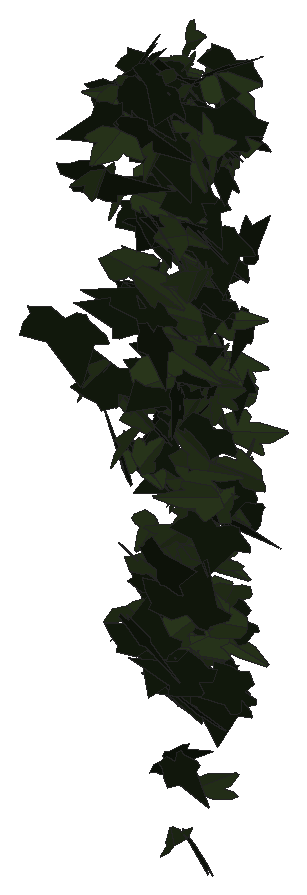
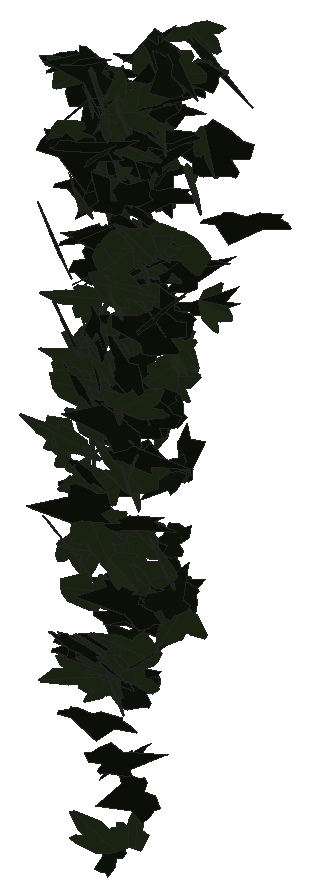
# SketchUp Ruby script. Lengths in millimetres.
U = 1.mm
M = Sketchup.active_model
def pt(a) = Geom::Point3d.new(a.map { |v| v * U })
def face(e, loops, mat)
  f = e.add_face(loops[0].map { |a| pt(a) })
  loops[1..].each { |l| e.add_face(l.map { |a| pt(a) }).erase! }
  f.material = f.back_material = mat if mat
  f
end
# faces: each face lists its corners as indices into pts; further lists are holes
def faces(e, pts, list, mat = nil) = list.each { |f| face(e, (f[0].is_a?(Array) ? f : [f]).map { |l| l.map { |i| pts[i] } }, mat) }
# xy, xz, yz: faces in a plane at the given z, y or x. An outline is a flat list of corners, or four numbers for a rectangle; further outlines are holes
def ring(l) = l.size == 4 ? [[l[0], l[1]], [l[2], l[1]], [l[2], l[3]], [l[0], l[3]]] : l.each_slice(2).to_a
def flat(e, list, mat, &to3) = list.each { |f| face(e, (f[0].is_a?(Array) ? f : [f]).map { |l| ring(l).map { |u, v| to3.(u, v) } }, mat) }
def xy(e, z, list, mat = nil) = flat(e, list, mat) { |x, y| [x, y, z] }
def xz(e, y, list, mat = nil) = flat(e, list, mat) { |x, z| [x, y, z] }
def yz(e, x, list, mat = nil) = flat(e, list, mat) { |y, z| [x, y, z] }
def lines(e, pts, list) = list.each { |a, b| e.add_line(pt(pts[a]), pt(pts[b])) }
# prism: a flat outline (further loops are holes) pulled along v
def prism(e, loops, v, mat = nil)
  f = face(e, loops, mat); d = Geom::Vector3d.new(v.map { |x| x * U })
  f.pushpull(f.normal.samedirection?(d) ? d.length : -d.length)
end
def box(e, o, s, mat = nil) = prism(e, [[o, [o[0] + s[0], o[1], o[2]], [o[0] + s[0], o[1] + s[1], o[2]], [o[0], o[1] + s[1], o[2]]]], [0, 0, s[2]], mat)
def at(x, y, z, deg = 0) = Geom::Transformation.translation(pt([x, y, z])) * Geom::Transformation.rotation(ORIGIN, Z_AXIS, deg.degrees)
def axes(o, x, y, z) = Geom::Transformation.new([*x, 0, *y, 0, *z, 0, *pt(o).to_a, 1])
def part(name) = M.definitions.add(name)
# library, detail: a bought-in or finely detailed component or shape, given as its bounding box
def library(name, o, s) = part(name).tap { |d| box(d.entities, o, s) }
def detail(e, o, s) = box(e.add_group.entities, o, s)
def put(e, d, t, mat = nil) = e.add_instance(d, t).tap { |i| i.material = mat if mat }
def group(e, t, mat = nil) = e.add_group.tap { |g| g.transformation = t; g.material = mat if mat }.entities
root = M.entities
M.materials.add("efeu1").color = [18, 25, 13]
M.materials.add("efeu2").color = [43, 57, 29]
c1 = part("ivyleaf_10")
p = [[0,12.8,-0.8],[-1.5,51.3,-10.9],[-4.9,51,-11.6],[-13.6,26.5,-7.3],[-13.2,15.9,-4.6],[-21.1,19.3,-7.2],
  [-29.5,16.3,-8.3],[-29.2,8.3,-6.2],[-19.7,-9.8,0.5],[-7.6,-13,4],[1,-12.2,5.8],[-0.4,51.1,-11.1],
  [-1.5,51.1,-10.9],[1,-12.4,5.9],[16.9,-12.4,3.5],[35.1,9.1,-5.1],[35,12.9,-6.1],[20.5,16.4,-4.9],
  [15.8,15,-3.8],[15.3,27.6,-7.1],[12.8,31.3,-7.8]]
faces(c1.entities,p,[[0,1,2,3,4,5,6,7,8,9,10],[11,12,0,13,14,15,16,17,18,19,20]],"efeu2")
c2 = part("ivyleaf_9")
p = [[39.1,54.8,31.7],[34.5,51.8,30.2],[-5.3,25.2,17.3],[-17.9,28.3,20.9],[-21.6,21.7,17],[-20.2,4.3,5.3],
  [-22.9,-0.3,2.5],[-17.1,-4,-0.6],[-2,-2.1,-1.2],[-0.7,-15.4,-10.1],[16.6,-22.3,-16.7],[21.1,-15.1,-12.5],
  [32.7,-10.7,-11],[46.1,-1.8,-6.6],[30.8,11.2,3.8]]
faces(c2.entities,p,[[0,1,2,3,4,5,6,7,8,9,10,11,12,13,14]],"efeu1")
put(root,c1,axes([3253.9,934.5,1390.3],[0.28843,0.04312,-0.8785],[1.25745,0.58285,0.14259],[1.10498,-0.67454,0.06705]))
put(root,c1,axes([3248.6,977.3,1386.9],[-0.36025,0.03868,0.8413],[1.53515,-0.23963,0.1925],[0.46091,0.82837,0.01641]))
put(root,c2,axes([3287.5,931.1,1234.8],[0.00435,-0.95208,0.10893],[0.11387,0.10886,0.95021],[-1.82026,0.00453,0.0597]))
put(root,c2,axes([3277.1,907.7,776.3],[1.0892,-0.78694,0.12747],[-0.13915,0.10444,0.97303],[-1.51082,-0.57695,0.00228]))
put(root,c1,axes([3291.6,962.2,1116.4],[1.27719,0.56046,0.4478],[-0.68997,-0.26417,0.87394],[1.17815,-0.76229,0.02637]))
put(root,c1,axes([3285.6,790.1,1475.8],[-0.46484,-1.03607,-0.08668],[0.02141,0.0864,-1.06443],[1.97862,-0.24434,-0.00884]))
put(root,c2,axes([3273,919,1588.6],[-0.4291,-0.87355,0.10052],[-0.05183,-0.09678,-0.90217],[1.67271,-0.22709,-0.00217]))
put(root,c2,axes([3281.5,876.4,1606.8],[0.34168,0.36068,0.93092],[0.51666,0.89258,-0.39818],[-1.82847,0.31961,0.06145]))
put(root,c2,axes([3265.6,884.9,987.3],[1.22662,-0.55899,-0.33011],[-0.47279,0.21739,-0.85315],[1.14149,0.69072,0.00136]))
put(root,c2,axes([3295.7,835.9,975.3],[0.02806,-0.50522,0.9314],[-0.00193,0.93148,0.50528],[-2.01663,-0.00792,0.01247]))
put(root,c1,axes([3299.6,879.7,1527.1],[-0.16158,0.22237,0.91702],[-1.11907,0.70764,-0.22604],[-1.40456,-0.58939,0.0746]))
put(root,c2,axes([3265.9,941.3,721.2],[0.65263,-0.85103,-0.29467],[-0.14747,0.28626,-0.91691],[1.70767,0.34997,0.03343]))
put(root,c1,axes([3287.3,900.9,857.4],[1.13215,-0.76866,-0.10225],[-0.11057,0.08433,-0.97195],[1.47166,0.59767,0.00564]))
put(root,c1,axes([3309.9,840.2,1594.3],[0.04476,0.06694,-1.05229],[-1.47456,-0.71285,-0.06266],[-1.36119,0.77442,0.03328]))
put(root,c2,axes([3311,992.6,552.1],[-0.28006,-0.04072,0.84102],[-1.52909,-0.24865,-0.15261],[0.47946,-0.81678,0.00453]))
put(root,c2,axes([3322.5,944.6,1028.3],[-1.09052,-0.28515,-0.64426],[-1.04808,-0.3367,0.6388],[-0.83635,0.79374,0.03953]))
put(root,c1,axes([3290.9,828.6,1425.4],[0.64577,-0.87683,-0.10025],[-0.03836,0.09968,-0.94004],[1.67922,0.33947,0.01708]))
put(root,c1,axes([3284.6,860.6,738.5],[-0.95757,-0.67439,-0.51289],[0.57513,0.41444,-0.84138],[1.50647,-0.58689,-0.0048]))
put(root,c2,axes([3274.9,887.2,1511.2],[-0.04256,-0.96485,-0.17622],[0.03285,0.17585,-0.96502],[1.86639,-0.0251,0.01297]))
put(root,c1,axes([3298.9,937.3,1019.6],[0.05472,0.6044,-0.66477],[-0.19068,0.66312,0.59856],[1.69927,0.05495,0.08858]))
put(root,c2,axes([3307.2,957.2,923.1],[-1.16527,-0.46556,0.47357],[-0.66857,-0.31958,-0.76835],[1.0726,-0.70499,0.03556]))
put(root,c1,axes([3296.2,821,1591],[0.65116,0.6651,-0.58723],[-0.60239,-0.49647,-0.74672],[-1.57749,0.46413,0.04275]))
put(root,c2,axes([3293.1,893.4,1564.3],[-1.0739,-0.73088,-0.0575],[0.06772,0.04517,-0.92335],[1.39367,-0.56538,0.00056]))
put(root,c2,axes([3275.2,889.6,1245.5],[1.73878,0.31637,0.12177],[0.22063,0.03738,-0.96683],[-0.60628,0.92093,-0.00259]))
put(root,c2,axes([3254,790.1,1452.3],[0.75139,0.00406,1.03661],[1.97244,-0.02493,-0.39462],[0.0416,1.10896,-0.01267]))
put(root,c1,axes([3300.8,925.7,1602.9],[-1.00619,-0.64272,-0.18805],[0.24655,0.13691,-0.83213],[1.25044,-0.54418,0.01275]))
put(root,c2,axes([3273.1,924,1076],[0.12484,0.02403,0.89967],[1.67971,0.17489,-0.06902],[-0.33534,0.88494,-0.01079]))
put(root,c1,axes([3304.7,973.1,861.9],[0.04218,-0.77693,0.45023],[0.00651,-0.45029,-0.7772],[1.70898,0.02089,-0.00815]))
put(root,c2,axes([3263,912.9,1216],[0.97935,-0.08083,0.79105],[1.48464,-0.13141,-0.52087],[0.29349,0.9345,-0.00482]))
put(root,c2,axes([3318.7,859.1,1636.9],[-0.74571,0.78825,-0.28221],[0.1694,-0.27061,-0.87941],[-1.58442,-0.39992,0.0388]))
put(root,c2,axes([3318.8,913.9,1399.8],[-1.60565,0.13671,-0.09247],[0.17432,-0.01285,-0.85466],[-0.2613,-0.84861,-0.00196]))
put(root,c2,axes([3298.6,916.5,1568.2],[1.35618,0.16441,0.50191],[-0.92402,-0.12791,0.73119],[0.39571,-0.86216,-0.01277]))
put(root,c1,axes([3291.3,944.5,1568.4],[0.64074,0.69136,0.43977],[0.31125,0.40918,-0.76847],[-1.52806,0.37325,0.02787]))
put(root,c2,axes([3323.4,819.4,1243.3],[-0.33755,-0.07382,1.03308],[-1.51767,-0.65909,-0.184],[1.25785,-0.81505,0.05523]))
put(root,c2,axes([3331.4,755.9,1587.4],[-1.42442,0.76046,-0.04851],[0.04929,-0.04257,-1.06692],[-1.44941,-0.74879,0.01139]))
put(root,c1,axes([3289.2,876.2,980],[1.06385,0.55203,0.36239],[0.49168,0.25413,-0.78562],[-1.15661,0.61579,-0.00065]))
put(root,c2,axes([3308.5,906,1248.9],[-1.124,0.21078,-0.58776],[1.00552,-0.2625,-0.625],[-0.63337,-0.79078,0.05081]))
put(root,c2,axes([3289.8,962.3,1152.2],[-0.15788,0.16375,0.96435],[0.41719,-0.94008,0.17849],[1.81426,0.23042,0.04288]))
put(root,c2,axes([3302.4,919.3,475.8],[-0.05073,0.44524,-0.77119],[-0.33069,0.75411,0.44138],[1.66221,0.16361,0.06427]))
put(root,c1,axes([3329.9,937.5,1342],[-0.61069,-0.20047,-0.81756],[-1.17253,-0.54029,0.37428],[-1.09171,0.69243,0.05535]))
put(root,c1,axes([3335,915.5,1564.5],[0.74949,0.03391,-0.76463],[-1.4523,-0.04923,-0.39519],[-0.11286,0.85867,0.00754]))
put(root,c1,axes([3299.9,908.4,1361.2],[1.36945,-0.49984,0.33483],[0.48733,-0.21791,-0.87559],[1.03612,0.76313,-0.03071]))
put(root,c1,axes([3314,826.4,1140.8],[0.20025,-0.96606,0.26786],[0.07402,-0.2652,-0.97173],[1.90654,0.11177,0.00959]))
put(root,c1,axes([3317.8,951.1,1594.5],[0.17462,-0.86742,-0.15138],[-0.0732,0.14811,-0.87198],[1.67423,0.09695,-0.02234]))
put(root,c2,axes([3315.5,943.5,1542.6],[-1.3993,-0.30438,-0.28687],[0.5207,0.08885,-0.79547],[0.60212,-0.7842,0.02123]))
put(root,c1,axes([3313.4,758,1181.1],[0.27822,-0.63831,0.81545],[0.27237,-0.80318,-0.65436],[1.95198,0.20305,-0.02492]))
put(root,c1,axes([3295.2,883.2,809.2],[-1.23284,-0.04385,-0.63204],[1.20276,0.01927,-0.64904],[0.08537,-0.90483,0.01681]))
put(root,c1,axes([3343.2,812.5,1085],[-0.79267,0.31669,-0.77791],[-1.17373,0.47414,0.52321],[1.08515,0.74418,-0.00231]))
put(root,c1,axes([3315.7,952.3,1630.6],[0.03877,-0.34001,-0.84093],[0.27102,0.83191,-0.33291],[1.70493,-0.12451,0.07205]))
put(root,c1,axes([3348.7,943.8,1282.5],[0.34788,0.12097,0.88791],[-1.59894,-0.29213,0.21275],[0.59333,-0.85817,0.05273]))
put(root,c2,axes([3326.3,879.2,977.8],[-1.68732,0.1692,0.27892],[0.50966,-0.08382,0.90205],[0.35459,0.92562,0.0307]))
put(root,c2,axes([3293,875.6,1051],[0.23174,-0.52444,0.80331],[0.57412,-0.74775,-0.5339],[1.73322,0.31781,0.06944]))
put(root,c1,axes([3309.3,926.4,1570],[-0.80304,-0.61089,-0.64139],[0.82938,0.47534,-0.73942],[1.46763,-0.60288,0.06691]))
put(root,c2,axes([3308.2,682.2,1290.5],[-0.73089,-0.96661,-0.43365],[0.33453,0.39674,-1.03999],[1.98836,-0.42206,0.01557]))
put(root,c1,axes([3291.7,832.5,1317.2],[-1.0633,-0.11437,-0.87816],[1.67338,0.05224,-0.56619],[0.20108,-1.0395,0.06816]))
put(root,c2,axes([3330.5,797.2,760.1],[-0.60982,0.46666,-0.8797],[-0.94036,0.72783,0.56607],[1.64548,0.58889,-0.00252]))
put(root,c2,axes([3300,824.2,1604.1],[-0.44666,-0.38765,-0.94717],[0.7948,0.8509,-0.45172],[1.77826,-0.47768,-0.03601]))
put(root,c2,axes([3311.4,947.6,1429.1],[-0.65615,-0.24268,0.89029],[1.49164,0.42465,0.41926],[-0.927,0.85507,0.04446]))
put(root,c1,axes([3294.6,927.7,701.9],[-0.52977,-0.18189,0.85888],[1.32472,0.50339,0.3322],[-1.01829,0.7495,-0.01467]))
put(root,c1,axes([3344.5,942.5,1313.6],[-1.39113,0.32766,-0.41608],[-0.73637,0.15387,0.80086],[0.68828,0.82688,0.01585]))
put(root,c2,axes([3346.1,750.4,1160.6],[-1.28897,-0.7664,0.23334],[0.29538,0.17425,1.02277],[-1.49584,0.69482,0.00089]))
put(root,c2,axes([3325.6,883,1073],[-0.59782,0.29431,-0.81585],[1.01079,-0.62073,-0.4284],[-1.305,-0.61561,0.04192]))
put(root,c1,axes([3358.5,924.7,1506.5],[0.33888,0.10545,-0.89522],[-1.7078,0.10744,-0.16582],[0.16301,0.90641,0.1238]))
put(root,c1,axes([3330.2,892.8,1314],[0.73888,-0.91558,-0.07321],[-0.04833,0.06875,-0.99448],[1.74742,0.38905,0.00345]))
put(root,c1,axes([3333.5,857.6,1618.6],[-0.74917,-0.98437,-0.06429],[0.04767,0.05922,-1.06016],[1.87684,-0.39443,0.00127]))
put(root,c2,axes([3312.2,947.3,1076.3],[0.07951,0.78909,-0.57645],[0.00785,0.57683,0.78991],[1.85984,-0.03617,0.02131]))
put(root,c2,axes([3311.3,886,763.5],[-0.72234,0.13403,0.72992],[1.18841,-0.38538,0.39544],[0.76328,0.72686,0.07507]))
put(root,c1,axes([3343,904.1,854.2],[-1.63168,-0.16884,0.1956],[-0.35684,-0.05992,-0.87353],[0.33839,-0.87732,0.02202]))
put(root,c1,axes([3345,887.6,872.3],[-0.71062,-0.63209,0.40984],[-0.40598,-0.34998,-0.73412],[1.37506,-0.42999,-0.00494]))
put(root,c1,axes([3338.9,908.1,1216.4],[-0.83833,-0.84952,0.01286],[-0.00161,-0.01404,-0.95691],[1.61698,-0.44045,0.00571]))
put(root,c2,axes([3331,928,1586.7],[-0.50278,-0.75655,0.4145],[-0.28888,-0.38598,-0.80122],[1.6162,-0.30434,-0.01427]))
put(root,c1,axes([3320.1,883.7,1191.9],[-0.55543,-0.32166,-0.72533],[0.93562,0.53333,-0.43431],[1.18535,-0.57169,0.00294]))
put(root,c1,axes([3329.7,904.6,641.8],[1.80385,-0.12497,0.0511],[-0.09009,0.03178,0.95567],[-0.24065,-0.94864,0.02528]))
put(root,c2,axes([3369.2,830.5,1267.1],[-0.90744,-0.03955,0.92066],[-1.6946,-0.24732,-0.47175],[0.45189,-1.00687,0.07972]))
put(root,c1,axes([3319.6,910.8,1252.4],[-0.9881,-0.63949,0.49513],[0.7293,0.32363,0.8198],[-1.35551,0.64028,0.08015]))
put(root,c1,axes([3336.6,951,1557.3],[-0.06939,-0.78211,0.47728],[0.17974,-0.47832,-0.7766],[1.73449,0.01828,0.09957]))
put(root,c2,axes([3321.8,855.5,1572.3],[0.3771,-0.83427,-0.33473],[-0.14545,0.32589,-0.85748],[1.70462,0.21236,0.00088]))
put(root,c1,axes([3331.8,828.5,1009.3],[0.18149,0.36128,-0.85355],[0.49089,0.81382,0.37328],[1.69432,-0.27448,-0.01672]))
put(root,c1,axes([3323.1,974.8,412.8],[-1.04981,-0.49762,0.50713],[0.73241,0.33044,0.74282],[-1.13669,0.6725,0.01026]))
put(root,c1,axes([3343.7,937.2,652],[0.77756,-0.74823,-0.27185],[-0.20243,0.25151,-0.85211],[1.50152,0.42137,0.0259]))
put(root,c2,axes([3359.4,861.7,1434.9],[-0.23841,-0.07301,1.05439],[-1.6678,-0.58643,-0.14472],[1.12458,-0.88518,0.00891]))
put(root,c1,axes([3327.9,835.3,1101.6],[-0.3131,-0.38781,-0.99947],[0.85259,0.89379,-0.42054],[1.85369,-0.4766,0.02461]))
put(root,c1,axes([3354.6,957.1,1453.5],[1.1528,-0.13981,0.59752],[-1.08137,0.18941,0.6203],[-0.44123,-0.82949,0.04093]))
put(root,c2,axes([3328.3,852.7,1399.8],[-0.5436,-0.79043,-0.46824],[0.25498,0.44927,-0.84013],[1.72979,-0.31462,-0.02331]))
put(root,c2,axes([3321.9,916.5,1074.1],[-0.29441,0.27045,0.80369],[0.60637,-0.73856,0.30986],[1.49563,0.35267,0.03258]))
put(root,c1,axes([3330.7,940.9,691.6],[-0.0142,-0.2389,-0.91823],[0.73177,0.83872,-0.22134],[1.65083,-0.37384,0.09021]))
put(root,c1,axes([3342.2,912.9,1574.8],[0.13573,-0.82464,0.38496],[0.16616,-0.37816,-0.82625],[1.72406,0.10137,0.04933]))
put(root,c2,axes([3326.6,874.5,1093.3],[-0.41023,-0.50578,-0.64108],[0.49383,0.58625,-0.54976],[1.47356,-0.33728,0.00577]))
put(root,c2,axes([3310.4,924.2,778.6],[0.07593,-0.18792,-0.90793],[1.55876,0.43308,-0.05365],[0.82707,-0.79897,0.18446]))
put(root,c1,axes([3336,940.2,1268.6],[0.49614,-0.57064,0.65422],[0.56498,-0.5833,-0.62707],[1.55261,0.39461,0.01913]))
put(root,c2,axes([3364.7,885.9,1551.4],[-1.46392,0.56427,-0.18567],[0.27723,-0.11532,-0.95394],[-1.09605,-0.78283,0.0067]))
put(root,c2,axes([3353.5,892.4,723.9],[-1.41179,-0.40603,0.51882],[0.88401,0.23175,0.84549],[-0.8892,0.87506,0.01682]))
put(root,c1,axes([3308.6,927.8,820.5],[0.32158,-0.13445,-1.04144],[1.71429,-0.52365,0.21374],[-1.02728,-0.91594,0.03067]))
put(root,c1,axes([3367.3,948.8,885.2],[-1.48699,0.01087,0.45029],[-0.85689,0.0071,-0.78139],[-0.02467,-0.90175,-0.00072]))
put(root,c1,axes([3346.3,885.1,370.7],[-0.26616,-0.72219,-0.46884],[-0.16708,-0.46055,0.73561],[-1.63017,0.16512,0.00115]))
put(root,c2,axes([3355.7,859.4,1166.3],[0.73945,-0.90706,0.23078],[-0.15563,0.21602,0.98673],[-1.77451,-0.39692,0.00963]))
put(root,c2,axes([3332.6,959.3,1513.1],[0.58905,-0.84912,-0.1149],[-0.0603,0.11074,-0.90373],[1.62965,0.31102,0.00809]))
put(root,c1,axes([3344.9,948.8,1163.8],[1.23336,-0.63701,0.0467],[-0.06177,0.03359,0.90871],[-1.21404,-0.64886,0.0012]))
put(root,c1,axes([3348.6,937.3,651.7],[-0.30742,-0.45799,-0.75211],[0.52941,0.69897,-0.48537],[1.59011,-0.32126,0.01619]))
put(root,c1,axes([3358.6,881.9,952.8],[0.3775,-0.98061,-0.08831],[-0.03776,0.08609,-1.00046],[1.87346,0.19933,-0.00237]))
put(root,c2,axes([3352.3,969.3,604.7],[-1.19521,-0.55094,-0.35137],[0.49077,0.23883,-0.83537],[1.14271,-0.67882,-0.00874]))
put(root,c2,axes([3339.9,852.7,1279.6],[0.26115,-0.88823,-0.26019],[-0.00294,0.26282,-0.898],[1.76152,0.13212,0.03707]))
put(root,c2,axes([3345.6,813.3,1417.7],[1.0119,-0.55021,-0.5356],[-0.67148,0.40357,-0.76481],[1.29797,0.63772,0.02189]))
put(root,c1,axes([3345.4,933.5,1158.8],[1.68299,-0.08577,0.18262],[0.34619,-0.01628,-0.88845],[0.16612,0.90281,0.00133]))
put(root,c2,axes([3360.5,801.7,728.9],[-1.34426,-0.31356,0.62057],[1.06892,0.26414,0.77272],[-0.78003,0.90234,-0.01055]))
put(root,c1,axes([3362.4,952,1611.8],[0.6455,-0.78851,-0.23172],[-0.13445,0.22178,-0.85808],[1.55836,0.34575,0.02195]))
put(root,c1,axes([3335.3,893.6,950.7],[-1.33824,-0.10498,0.70648],[1.32856,0.10878,0.71094],[-0.28766,0.99081,-0.0032]))
put(root,c2,axes([3345.8,886.9,638.9],[-0.30776,-0.63797,-0.51265],[0.25371,0.49505,-0.65811],[1.53682,-0.20949,0.00598]))
put(root,c2,axes([3368.4,871.3,1098],[0.4215,0.16104,0.80389],[-1.32508,-0.40278,0.27249],[0.82396,-0.73011,0.02699]))
put(root,c2,axes([3348.7,911.1,1032.5],[0.66556,0.64701,0.51065],[-0.48178,-0.4436,0.73541],[1.4929,-0.4316,0.00967]))
put(root,c2,axes([3390.1,960.3,1490.9],[-1.47426,-0.66786,-0.13671],[-0.17636,-0.10187,1.02265],[-1.2854,0.77997,0.01649]))
put(root,c1,axes([3332.1,951.6,1094],[0.14133,-0.04856,-0.90261],[1.30628,-0.58629,0.08801],[-1.11945,-0.69027,-0.01125]))
put(root,c1,axes([3367.1,723.7,1590.3],[1.15698,0.54771,-0.47669],[-0.66918,-0.3219,-0.81825],[-1.20908,0.70226,-0.00328]))
put(root,c2,axes([3325,792.2,1562.3],[0.6749,-0.03639,-0.85389],[1.37565,0.5061,0.2786],[0.868,-0.77379,0.22238]))
put(root,c2,axes([3364.5,848.9,703],[-1.15194,-0.76493,0.00311],[-0.00301,-0.00272,-0.97543],[1.45582,-0.60527,0.00045]))
put(root,c2,axes([3329.2,883.9,612.1],[0.99319,-0.47308,0.56669],[0.85274,-0.34856,-0.70359],[1.11657,0.68701,0.03326]))
put(root,c2,axes([3324.8,909.6,1337.2],[1.42316,-0.43328,0.56399],[0.89331,-0.31418,-0.86369],[1.01694,0.88235,-0.03059]))
put(root,c2,axes([3355.1,848.1,1616.2],[-0.33146,-0.8045,0.71653],[-0.1516,-0.71423,-0.82128],[2.04476,-0.18336,0.05526]))
put(root,c2,axes([3352.9,879.7,504],[0.44572,-0.67682,-0.46544],[-0.25658,0.44576,-0.71603],[1.54212,0.26979,0.01539]))
put(root,c2,axes([3345.4,961.4,1218.7],[-0.2195,-0.0041,-0.98294],[1.75243,-0.34684,-0.10659],[-0.65476,-0.92692,0.04423]))
put(root,c1,axes([3368.7,757.6,1093.9],[0.25397,-0.81199,0.58918],[0.17568,-0.58191,-0.82288],[1.90123,0.16223,-0.00267]))
put(root,c2,axes([3395.3,972.5,711.4],[-1.65827,0.21897,0.14719],[-0.27284,0.03346,-0.8984],[-0.42155,-0.88302,0.00245]))
put(root,c1,axes([3345.3,936,675.2],[1.35679,-0.10552,-0.53238],[1.03158,0.09334,0.70731],[-0.05299,-0.88484,0.1381]))
put(root,c1,axes([3409.7,834.4,1265.2],[-0.28217,-0.02139,1.06528],[-1.94413,-0.30301,-0.14825],[0.57669,-1.03199,0.02145]))
put(root,c1,axes([3377,856.4,1492.1],[0.12815,-0.27016,-0.88247],[-0.05068,0.88387,-0.27262],[1.75572,0.04524,0.05654]))
put(root,c1,axes([3375.4,871.7,1447.7],[-0.02591,-0.86994,0.34595],[0.09743,-0.34616,-0.86845],[1.77911,0.00628,0.0526]))
put(root,c1,axes([3362.8,989.4,1447.1],[1.09016,-0.61177,0.40413],[0.54833,-0.28378,-0.83794],[1.28318,0.64101,0.01473]))
put(root,c1,axes([3379.2,874.7,1319.9],[-1.48448,0.3281,0.11887],[-0.21269,0.04089,-0.84617],[-0.62917,-0.78794,0.00559]))
put(root,c2,axes([3350.9,918.8,354.5],[0.81286,-0.24571,-0.70668],[1.15894,-0.35862,0.49272],[-0.82732,-0.74378,-0.00412]))
put(root,c2,axes([3389.3,815.7,1417.8],[0.67839,0.698,-0.69959],[-0.62644,-0.61739,-0.78369],[-1.77344,0.48509,0.00921]))
put(root,c2,axes([3352.7,879.7,670.5],[0.32961,-0.53157,0.6471],[0.42799,-0.607,-0.55881],[1.53527,0.28334,0.01686]))
put(root,c2,axes([3362.2,838.1,1531.5],[-0.29916,-0.92378,-0.4774],[0.21493,0.4648,-0.93658],[1.96733,-0.19125,0.02973]))
put(root,c1,axes([3346.1,824.3,1438.6],[0.44248,0.16499,0.98686],[1.35782,0.68301,-0.28227],[-1.33512,0.7493,0.04]))
put(root,c1,axes([3375,806.8,1540.6],[0.10409,-0.78668,0.55718],[0.38233,-0.53653,-0.77724],[1.79443,0.15995,0.13328]))
put(root,c2,axes([3355.9,940.4,1505.6],[1.56632,-0.38854,-0.39815],[0.69178,-0.16267,0.91007],[-0.80154,-0.89966,0.0074]))
put(root,c1,axes([3367,893.1,743.9],[1.70353,0.30491,-0.29401],[0.50165,0.1371,0.94463],[0.63105,-0.93211,0.04277]))
put(root,c2,axes([3384.9,808.2,1165.3],[-0.80305,-0.70639,0.65777],[-0.55207,-0.59189,-0.82171],[1.75209,-0.51027,0.04257]))
put(root,c2,axes([3399.9,894.4,1568.6],[0.45965,0.51878,-0.876],[-0.63252,-0.81081,-0.57181],[-1.83148,0.41022,-0.02237]))
put(root,c2,axes([3392.5,955.7,1502],[0.88332,0.58606,-0.43426],[-0.54601,-0.32656,-0.74734],[-1.27633,0.5453,0.01917]))
put(root,c2,axes([3371,958.2,1576.2],[0.72681,-0.74963,-0.42336],[-0.40378,0.36692,-0.84106],[1.58797,0.4364,-0.02009]))
put(root,c1,axes([3416.6,945.2,1099],[0.23667,0.08332,0.96406],[-1.53163,-0.53082,0.14968],[1.02263,-0.81431,0.00107]))
put(root,c1,axes([3357.8,974,667.1],[0.67703,0.29059,0.78873],[1.21109,0.46647,-0.45887],[-1.0452,0.72873,-0.02079]))
put(root,c1,axes([3376.6,841,740.1],[0.30331,0.34549,-0.88816],[0.73767,0.79915,0.38041],[1.65694,-0.41902,-0.00678]))
put(root,c1,axes([3386.8,937.6,1040.9],[-1.3545,0.50311,0.24217],[0.35199,-0.15779,0.87131],[1.00268,0.73503,0.02128]))
put(root,c2,axes([3374.6,924.3,1607.2],[-0.03741,0.77556,-0.47178],[-0.00972,0.47179,0.77579],[1.72766,0.01945,-0.00585]))
put(root,c1,axes([3391.6,904.1,1094.1],[-1.0262,-0.71453,-0.14688],[0.19224,0.10775,-0.89501],[1.37495,-0.54836,0.01551]))
put(root,c2,axes([3398.6,990.1,890],[-1.53585,0.35413,-0.49466],[0.84122,-0.22332,-0.88095],[-0.79555,-0.9198,0.02344]))
put(root,c2,axes([3365.3,763.3,782.8],[1.18103,-0.77596,0.01837],[0.02162,-0.01443,-0.99358],[1.47707,0.62065,-0.00014]))
put(root,c2,axes([3413.9,896.4,1149.1],[-0.36553,0.11433,-1.0557],[-1.6713,0.58607,0.22323],[1.13624,0.89884,-0.01127]))
put(root,c2,axes([3416.1,848.4,1450.6],[-0.98289,-0.87799,-0.04218],[-0.0275,-0.04044,1.01859],[-1.6727,0.51658,0.00804]))
put(root,c1,axes([3398.3,914.9,1019.4],[0.51116,-0.72193,-0.55385],[-0.15379,0.55627,-0.76426],[1.72489,0.26354,0.09599]))
put(root,c1,axes([3398.1,851.3,1111.5],[-0.12164,-0.95484,0.36693],[-0.0135,-0.36722,-0.95684],[1.94677,-0.06221,0.01629]))
put(root,c1,axes([3372,787,1168.2],[0.439,0.19503,-1.08225],[1.25237,0.86149,0.2955],[1.67686,-0.69447,0.06264]))
put(root,c1,axes([3396,896.4,1153.7],[0.2057,-0.30144,0.9377],[-0.44965,0.90785,0.31907],[-1.81984,-0.25839,0.02715]))
put(root,c2,axes([3415.2,900.7,652.7],[-0.5546,0.81658,0.2578],[-0.18033,0.2399,-0.86698],[-1.61971,-0.30631,0.00825]))
put(root,c1,axes([3416.7,957.2,1507.1],[0.32459,0.25103,-0.81469],[-1.34302,-0.42459,-0.27856],[-0.91032,0.71592,0.12047]))
put(root,c1,axes([3400.4,919.9,1472.2],[-0.01559,-0.90582,0.37714],[0.01363,-0.3772,-0.9058],[1.86736,-0.00481,0.00976]))
put(root,c1,axes([3407.6,884.4,1185.5],[-0.31204,0.95139,-0.28525],[-0.15804,0.27497,0.96483],[1.8837,0.18067,0.0337]))
put(root,c2,axes([3417.6,923.2,1329.4],[-0.08468,-0.80674,-0.57929],[-0.07328,-0.57804,0.80795],[-1.8888,0.05859,-0.00537]))
put(root,c1,axes([3366.8,836,1402.9],[-0.29172,-0.01895,1.02335],[1.92141,-0.1731,0.14801],[0.32061,1.02018,0.04412]))
put(root,c2,axes([3394.9,902.7,1268.9],[-0.31698,-0.8812,0.23032],[-0.0742,-0.22703,-0.89679],[1.73185,-0.17101,0.00373]))
put(root,c2,axes([3386.1,868.3,1438.7],[-0.65686,-0.49854,-0.67397],[0.92371,0.47546,-0.60023],[1.3009,-0.58932,0.08589]))
put(root,c2,axes([3399.7,952.3,1624],[-0.61785,-0.82684,0.07489],[-0.03808,-0.0726,-0.88826],[1.57963,-0.32516,0.00788]))
put(root,c1,axes([3410.5,861.6,1537.9],[1.91722,-0.17015,0.32042],[-0.5994,0.05924,1.02162],[-0.34272,-1.05544,0.00569]))
put(root,c2,axes([3407.6,923.8,1247.7],[-0.40501,-0.20613,0.86124],[-0.56346,-0.81823,-0.26899],[1.58842,-0.34281,0.12418]))
put(root,c1,axes([3383.2,896.2,851.7],[-1.23118,-0.18161,-0.77389],[1.42917,0.1877,-0.67175],[0.4963,-0.99104,0.0146]))
put(root,c1,axes([3407.6,882.5,1504.6],[1.1255,-0.71726,0.00658],[0.00803,-0.00505,-0.92962],[1.36512,0.59139,0.00004]))
put(root,c1,axes([3413.9,906.2,1570.2],[0.38066,-0.8185,-0.31435],[-0.09797,0.31091,-0.84229],[1.66583,0.20532,0.0223]))
put(root,c2,axes([3423,889,1275.2],[-0.29793,-0.10174,-0.85456],[0.07137,-0.86856,0.09653],[-1.63632,-0.01936,0.1598]))
put(root,c1,axes([3434.5,902.9,747.3],[0.04709,0.1004,0.93046],[-1.11652,-0.72354,0.09367],[1.38774,-0.58554,0.04379]))
put(root,c2,axes([3375.9,927.3,901.5],[1.42612,-0.22892,0.45876],[0.83137,-0.14027,-0.7835],[0.51085,0.86734,-0.00563]))
put(root,c1,axes([3392.8,905.5,940.6],[-1.29062,-0.01227,-0.5911],[1.12375,0.03186,-0.67806],[0.05743,-0.89902,-0.01596]))
put(root,c1,axes([3439.2,822.8,1059.8],[-0.10751,0.1057,-0.9716],[-1.22452,0.72856,0.11667],[1.40014,0.64529,0.02743]))
put(root,c2,axes([3420.8,785.1,1402.5],[0.49573,-0.80529,0.40639],[-0.09795,0.40904,0.84353],[-1.71394,-0.25629,0.06934]))
put(root,c2,axes([3384.1,816.6,1190.2],[-0.6069,0.14608,1.05736],[1.66752,-0.59447,0.34637],[1.1603,0.93075,0.05527]))
put(root,c1,axes([3382.8,867,997.7],[-0.57774,-0.12857,0.91473],[1.58819,0.37473,0.3296],[-0.75389,0.88796,-0.00665]))
put(root,c2,axes([3405.8,950.6,1123.1],[-1.03256,0.10059,-0.7366],[1.38345,-0.11945,-0.55171],[-0.29672,-0.90701,-0.00903]))
put(root,c2,axes([3403.5,855.5,1397.9],[1.72063,-0.29541,-0.45534],[-0.79748,0.18244,-0.95031],[0.65662,0.99569,0.03903]))
put(root,c1,axes([3385.7,769,1344.3],[-0.24361,0.06819,-0.96168],[1.42361,-0.60503,-0.14246],[-1.15762,-0.7584,0.02718]))
put(root,c1,axes([3399.7,940.2,1145.8],[1.33875,0.4508,0.34881],[0.54474,0.19977,-0.83538],[-0.93813,0.75932,0.01269]))
put(root,c2,axes([3406.8,968.8,1316.6],[-0.34158,0.75672,0.6815],[-0.01839,-0.69323,0.76721],[1.93807,0.12679,0.12739]))
put(root,c1,axes([3394.8,908.8,1115.1],[-1.17274,0.08013,0.74335],[1.39618,-0.12115,0.62117],[0.27468,0.95791,0.01638]))
put(root,c2,axes([3409.7,907.3,1548],[-0.89414,0.10038,-0.74397],[1.34579,-0.23553,-0.47832],[-0.47976,-0.84778,0.0448]))
put(root,c2,axes([3418.8,954.1,1208.7],[-1.1169,0.32547,-0.74128],[1.24534,-0.34843,-0.67101],[-0.9073,-0.87891,-0.00849]))
put(root,c2,axes([3417.8,820.5,796.9],[-1.7126,0.28307,0.57308],[1.01252,-0.21683,0.94246],[0.67427,1.04458,0.04033]))
put(root,c1,axes([3435.8,777.6,1434.5],[0.886,-0.54752,-0.60802],[-0.75246,0.46193,-0.71867],[1.36335,0.61076,-0.00152]))
put(root,c1,axes([3399.5,923.2,1602.2],[1.1019,0.55131,0.53461],[0.74966,0.36155,-0.79943],[-1.25467,0.70021,-0.00814]))
put(root,c2,axes([3448,803.4,703.1],[-0.37804,0.01983,0.8844],[-1.60807,-0.27271,-0.18366],[0.49864,-0.86443,0.07823]))
put(root,c2,axes([3416,892.1,633.5],[-1.38459,-0.27777,-0.57547],[1.00629,0.22803,-0.77848],[0.68294,-0.89913,-0.01965]))
put(root,c1,axes([3415.1,878.8,855.4],[-1.35218,-0.38215,0.26134],[0.45217,0.1099,0.80659],[-0.75625,0.749,0.01499]))
put(root,c1,axes([3397.6,852.3,1520.1],[0.90469,-0.25127,0.8398],[1.35059,-0.45052,-0.53647],[0.97938,0.85338,-0.03595]))
put(root,c2,axes([3422.9,924,966.9],[-1.39696,-0.01656,-0.54895],[1.04469,-0.05184,-0.73239],[-0.0339,-0.91511,0.05142]))
put(root,c1,axes([3414.6,864.4,1166.1],[-0.55812,-0.4429,-0.82357],[0.84153,0.69486,-0.53112],[1.56818,-0.53051,-0.0081]))
put(root,c2,axes([3412.7,806.5,1154.9],[0.00009,-0.00768,-0.94566],[1.33549,-0.63397,0.00518],[-1.20661,-0.70168,0.00567]))
put(root,c2,axes([3400.9,777.6,880.7],[-0.0491,0.1064,0.9827],[0.76635,-0.89664,0.10765],[1.71804,0.403,-0.01994]))
put(root,c2,axes([3425.5,878.2,910.8],[-1.20081,-0.62103,-0.26762],[0.33982,0.20004,-0.88515],[1.24135,-0.65551,-0.01658]))
put(root,c2,axes([3413.2,898.8,1483.2],[-0.00651,-0.72917,0.49874],[0.05009,-0.49861,-0.7288],[1.68059,0.01204,0.02365]))
put(root,c2,axes([3465.1,884.2,1560.4],[-0.61168,0.10096,1.00271],[-1.91789,-0.04337,-0.31863],[0.02037,-1.05206,0.10936]))
put(root,c1,axes([3402.2,910.9,1229.2],[0.19818,-0.07878,-0.89708],[1.42001,0.51321,0.04154],[0.95968,-0.74311,0.12379]))
put(root,c1,axes([3453.7,820.6,995.7],[0.40735,0.12735,-0.91404],[-1.56462,-0.40005,-0.24824],[-0.79809,0.84926,0.02013]))
put(root,c1,axes([3428.7,936.8,986],[0.53189,-0.67877,0.53629],[-0.39594,0.49431,0.73404],[-1.59807,-0.34839,-0.00337]))
put(root,c2,axes([3432.8,858.8,1079.6],[-1.53408,-0.19675,-0.30461],[0.56055,0.07791,-0.8297],[0.40261,-0.85816,-0.00548]))
put(root,c1,axes([3422.9,875.7,812.3],[-0.07253,0.8763,0.22752],[-0.02083,0.22726,-0.87713],[-1.72295,-0.03964,0.00103]))
put(root,c2,axes([3411.2,755.2,1273],[-0.76034,0.01616,-0.88873],[1.66694,-0.15899,-0.39661],[-0.28847,-0.96134,0.05066]))
put(root,c1,axes([3434.2,816.8,1349.8],[-0.70892,-0.96651,-0.04003],[0.0268,0.03748,-1.03581],[1.84085,-0.37276,-0.00034]))
put(root,c2,axes([3454.9,898.4,649.2],[-0.92335,-0.24244,0.72749],[-1.24556,-0.31773,-0.54234],[0.76058,-0.81466,-0.00498]))
put(root,c1,axes([3396.9,961.9,1023.4],[0.72182,-0.1107,-0.83626],[1.60256,-0.00548,0.38261],[-0.09659,-0.91823,0.09854]))
put(root,c1,axes([3464.4,911,995.1],[-0.28126,0.02089,0.9241],[-1.75872,0.01827,-0.14819],[-0.04061,-0.93566,0.01774]))
put(root,c1,axes([3429.7,878.8,945.3],[0.35047,0.16397,-0.89404],[0.31581,0.89081,0.19755],[1.70084,-0.19919,0.14754]))
put(root,c1,axes([3441.7,891.5,811.1],[-0.96712,-0.73665,0.12773],[-0.13664,-0.10564,-0.89492],[1.41633,-0.5132,0.00088]))
put(root,c1,axes([3438.3,831.6,1342.9],[0.46238,-0.93196,-0.3254],[-0.06814,0.32657,-0.96204],[1.87747,0.24137,0.04522]))
put(root,c2,axes([3423.1,871.9,1390.8],[-0.80674,-0.91668,-0.39818],[0.33118,0.35821,-1.00992],[1.87306,-0.45816,0.00707]))
put(root,c1,axes([3398.3,808.7,1218.5],[0.63935,0.09789,0.93206],[1.72259,0.22299,-0.34964],[-0.46275,0.96534,-0.01375]))
